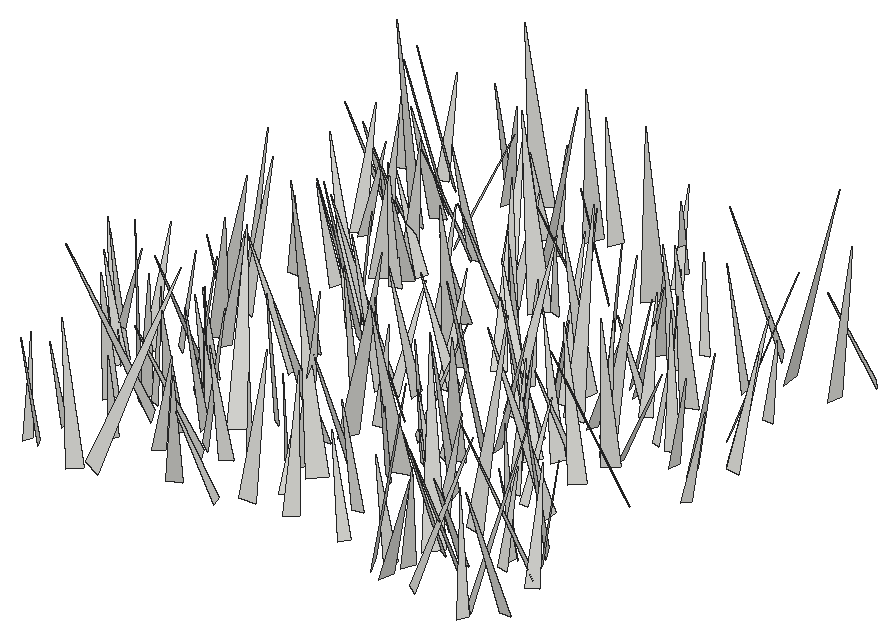
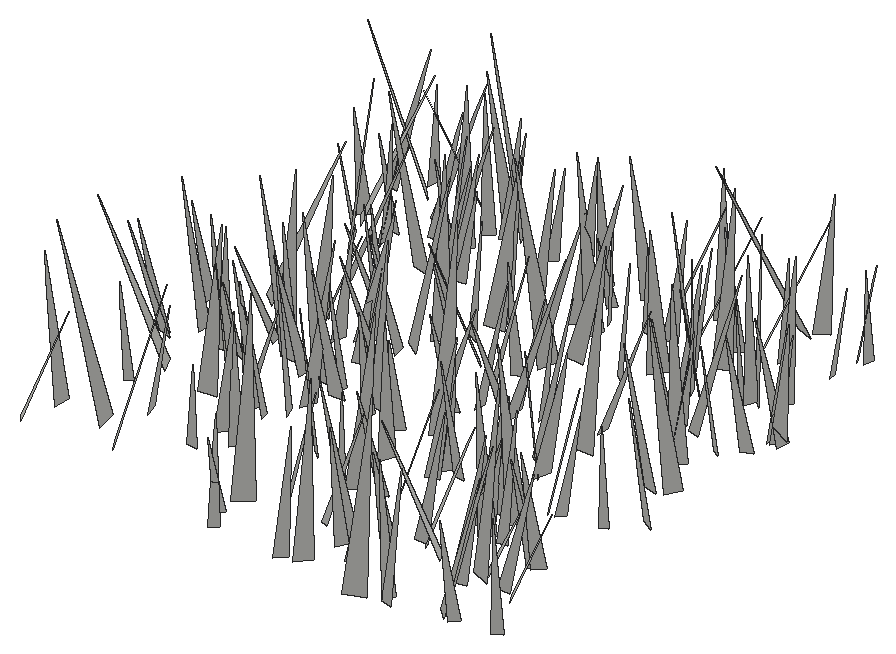
# SketchUp Ruby script. Lengths in inches.
U = 1.inch
M = Sketchup.active_model
def pt(a) = Geom::Point3d.new(a.map { |v| v * U })
def face(e, loops, mat)
  f = e.add_face(loops[0].map { |a| pt(a) })
  loops[1..].each { |l| e.add_face(l.map { |a| pt(a) }).erase! }
  f.material = f.back_material = mat if mat
  f
end
# faces: each face lists its corners as indices into pts; further lists are holes
def faces(e, pts, list, mat = nil) = list.each { |f| face(e, (f[0].is_a?(Array) ? f : [f]).map { |l| l.map { |i| pts[i] } }, mat) }
# xy, xz, yz: faces in a plane at the given z, y or x. An outline is a flat list of corners, or four numbers for a rectangle; further outlines are holes
def ring(l) = l.size == 4 ? [[l[0], l[1]], [l[2], l[1]], [l[2], l[3]], [l[0], l[3]]] : l.each_slice(2).to_a
def flat(e, list, mat, &to3) = list.each { |f| face(e, (f[0].is_a?(Array) ? f : [f]).map { |l| ring(l).map { |u, v| to3.(u, v) } }, mat) }
def xy(e, z, list, mat = nil) = flat(e, list, mat) { |x, y| [x, y, z] }
def xz(e, y, list, mat = nil) = flat(e, list, mat) { |x, z| [x, y, z] }
def yz(e, x, list, mat = nil) = flat(e, list, mat) { |y, z| [x, y, z] }
def lines(e, pts, list) = list.each { |a, b| e.add_line(pt(pts[a]), pt(pts[b])) }
# prism: a flat outline (further loops are holes) pulled along v
def prism(e, loops, v, mat = nil)
  f = face(e, loops, mat); d = Geom::Vector3d.new(v.map { |x| x * U })
  f.pushpull(f.normal.samedirection?(d) ? d.length : -d.length)
end
def box(e, o, s, mat = nil) = prism(e, [[o, [o[0] + s[0], o[1], o[2]], [o[0] + s[0], o[1] + s[1], o[2]], [o[0], o[1] + s[1], o[2]]]], [0, 0, s[2]], mat)
def at(x, y, z, deg = 0) = Geom::Transformation.translation(pt([x, y, z])) * Geom::Transformation.rotation(ORIGIN, Z_AXIS, deg.degrees)
def axes(o, x, y, z) = Geom::Transformation.new([*x, 0, *y, 0, *z, 0, *pt(o).to_a, 1])
def part(name) = M.definitions.add(name)
# library, detail: a bought-in or finely detailed component or shape, given as its bounding box
def library(name, o, s) = part(name).tap { |d| box(d.entities, o, s) }
def detail(e, o, s) = box(e.add_group.entities, o, s)
def put(e, d, t, mat = nil) = e.add_instance(d, t).tap { |i| i.material = mat if mat }
def group(e, t, mat = nil) = e.add_group.tap { |g| g.transformation = t; g.material = mat if mat }.entities
root = M.entities
c1 = part("fur_instance\#9")
p = [[0.8125,0,1.79],[0.67,-0.02,1.48],[0,-0.11,0],[0,0.11,0]]
faces(c1.entities,p,[[0,1,2,3]])
put(root,c1,axes([502.1875,404.34,-21.66],[2.0816,-3.74764,1.04429],[-3.88491,-2.06538,0.3318],[-0.20701,1.076,4.27408]))
put(root,c1,axes([503.84,370.23,-21.66],[3.17127,-3.30736,3.04126],[-3.82504,-3.9403,-0.2965],[-2.35731,1.94429,4.57249]))
put(root,c1,axes([504.64,399.73,-21.66],[-3.58425,-2.16039,0.18109],[-2.16614,3.55434,-0.47063],[-0.08907,0.49634,4.15845]))
put(root,c1,axes([504.66,370.01,-21.66],[-5.03296,-0.41167,1.23228],[-0.52474,5.15421,-0.42127],[1.18855,0.5323,5.03216]))
put(root,c1,axes([503.76,385.25,-21.66],[2.58353,5.00263,1.49189],[5.09313,-2.78069,0.50442],[-1.14546,-1.08079,5.60772]))
put(root,c1,axes([504.62,369.6,-21.66],[-3.50037,2.65675,1.28484],[2.86731,3.53339,0.50538],[0.69832,-1.19104,4.36526]))
put(root,c1,axes([503.45,370.17,-21.66],[4.85484,-0.93426,0.93937],[-1.01134,-4.91828,0.33525],[-0.85583,0.51221,4.93253]))
put(root,c1,axes([504.86,372.58,-21.66],[-0.99114,4.85366,1.48422],[5.00835,1.18049,-0.51592],[0.82303,-1.33855,4.92689]))
put(root,c1,axes([505.76,399.13,-21.66],[0.4513,-4.46287,0.47479],[-4.46772,-0.49211,-0.3789],[-0.42669,0.43236,4.4696]))
put(root,c1,axes([507.15,404.4375,-21.66],[2.82941,3.82153,3.56935],[4.50896,-3.83832,0.53527],[-2.64833,-2.45217,4.72474]))
put(root,c1,axes([506.2,356.96,-21.66],[-3.76859,1.24193,1.36163],[1.17189,4.00702,-0.41131],[1.42236,-0.01087,3.94658]))
put(root,c1,axes([505.79,395.09,-21.66],[-2.49427,4.27012,1.59064],[4.35584,2.76683,-0.59729],[1.33819,-1.04698,4.90903]))
put(root,c1,axes([505.79,404.8,-21.66],[2.7326,-2.75522,2.01665],[-3.2693,-2.85632,0.52755],[-0.98478,1.83723,3.84448]))
put(root,c1,axes([507.12,357.09,-21.66],[-3.57369,-1.9669,1.0397],[-2.0892,3.64317,-0.28897],[0.76478,0.76131,4.06896]))
put(root,c1,axes([505.91,387.55,-21.66],[0.58274,-3.68979,0.92218],[-3.78198,-0.46356,0.53511],[0.40205,0.98748,3.697]))
put(root,c1,axes([506.95,360.17,-21.66],[-3.35519,-0.75879,1.11745],[-0.66434,3.53232,0.40387],[1.17606,-0.1694,3.41613]))
put(root,c1,axes([508.16,397.96,-21.66],[-3.2308,-2.41105,0.08917],[-2.40238,3.20101,-0.49122],[-0.22293,0.4467,4.00124]))
put(root,c1,axes([505.3,380.38,-21.66],[5.59181,-3.37862,1.09906],[-3.46581,-5.63815,0.30113],[-0.78177,0.82912,6.52631]))
put(root,c1,axes([506.53,374.04,-21.66],[2.33806,3.32528,1.40975],[3.5899,-2.32407,-0.47188],[-0.3968,-1.43269,4.03749]))
put(root,c1,axes([506.39,395.07,-21.66],[3.89931,-1.45547,0.98195],[-1.58431,-3.9476,0.44006],[-0.75669,0.76505,4.13877]))
put(root,c1,axes([507.09,365.31,-21.66],[4.37094,-3.26497,1.75227],[-3.26747,-4.6741,-0.55863],[-1.74761,0.57306,5.42707]))
put(root,c1,axes([506.81,381.15,-21.66],[1.78136,5.8506,1.71123],[6.09225,-1.76893,-0.29408],[-0.20572,-1.72409,6.10871]))
put(root,c1,axes([508.73,401.61,-21.66],[-4.07714,-4.72232,1.18622],[-4.85623,4.056,-0.54439],[0.3528,1.25658,6.21506]))
put(root,c1,axes([507.76,377.96,-21.66],[-3.40624,-2.616,1.08161],[-2.59295,3.56228,0.44999],[1.13575,0.28715,4.27123]))
put(root,c1,axes([508.3125,398.65,-21.66],[-2.90002,-7.26429,3.03178],[-7.85451,2.88308,-0.60516],[0.51793,3.0479,7.79832]))
put(root,c1,axes([511.03,365.12,-21.66],[-6.73685,-3.71008,0.0403],[-3.70619,6.73292,0.28887],[0.17463,-0.23362,7.68547]))
put(root,c1,axes([508.9375,366.28,-21.66],[4.24793,5.0228,3.04998],[5.34423,-4.86703,0.57187],[-2.44337,-1.91294,6.55335]))
put(root,c1,axes([509.41,388.08,-21.66],[-3.58724,1.8714,1.40372],[2.1412,3.66165,0.59026],[0.94225,-1.19623,4.00275]))
put(root,c1,axes([508.99,400.3,-21.66],[1.67149,-5.33301,0.8085],[-5.34441,-1.75188,-0.5067],[-0.72935,0.6152,5.5658]))
put(root,c1,axes([507.59,376.98,-21.66],[3.73697,-5.4189,0.58942],[-5.45085,-3.71358,0.41766],[0.01126,0.72231,6.56925]))
put(root,c1,axes([509.49,372.86,-21.66],[-2.17037,-5.72704,0.1674],[-5.69455,2.17595,0.61228],[0.63178,-0.0613,6.09382]))
put(root,c1,axes([509,366.91,-21.66],[5.28351,-1.61661,1.62366],[-1.56193,-5.52709,-0.42043],[-1.67632,0.05465,5.50927]))
put(root,c1,axes([508.7,376.28,-21.66],[4.80209,-1.99507,1.20954],[-2.10711,-4.89697,0.2883],[-1.00169,0.73669,5.19204]))
put(root,c1,axes([510,366.68,-21.66],[1.76175,3.91399,1.38102],[4.01071,-1.99148,0.5277],[-1.06803,-1.02224,4.25965]))
put(root,c1,axes([510.51,388.11,-21.66],[-3.88391,-3.01754,1.00768],[-2.99103,4.00531,0.46572],[1.08383,0.24005,4.89626]))
put(root,c1,axes([510.1,393.9,-21.66],[0.02895,-4.95019,0.58964],[-4.94989,0.0415,0.59139],[0.59214,0.58889,4.91483]))
put(root,c1,axes([511.05,372.22,-21.66],[0.17752,-3.57602,1.3313],[-3.7929,-0.31113,-0.32997],[-0.41733,1.30655,3.56518]))
put(root,c1,axes([511.4,355.79,-21.66],[-3.51075,4.42455,2.16586],[4.8357,3.60279,0.47842],[0.94002,-2.00904,5.62789]))
put(root,c1,axes([511.19,405.79,-21.66],[-1.65824,-4.82946,1.36253],[-4.95542,1.80194,0.35604],[0.78993,1.16588,5.09379]))
put(root,c1,axes([510.89,360.84,-21.66],[3.12862,-2.29976,0.97047],[-2.27,-3.26853,-0.42753],[-1.03819,0.21622,3.85932]))
put(root,c1,axes([511.2,369.73,-21.66],[3.52114,3.87417,1.40413],[3.91467,-3.72163,0.45161],[-1.28689,-0.72073,5.21571]))
put(root,c1,axes([514.11,384.43,-21.66],[-6.63605,2.7216,0.19643],[2.70208,6.62626,-0.52374],[0.38006,0.41041,7.15332]))
put(root,c1,axes([513.33,392.98,-21.66],[-4.0044,1.49429,0.5536],[1.5481,4.00291,0.3933],[0.37782,-0.56428,4.25599]))
put(root,c1,axes([511.1,390.97,-21.66],[5.02607,-4.57327,2.19343],[-4.92834,-5.13329,0.59007],[-1.19892,1.92923,6.76964]))
put(root,c1,axes([512.8125,390.61,-21.66],[-0.34045,4.62028,2.07312],[5.05885,0.21591,0.34957],[-0.23002,-2.08976,4.6196]))
put(root,c1,axes([511.52,405.07,-21.66],[4.68677,-2.0034,0.66372],[-1.95488,-4.73014,-0.47351],[-0.79535,-0.17932,5.07496]))
put(root,c1,axes([511.71,393.625,-21.66],[3.13383,-5.16211,1.39491],[-5.34355,-3.08346,0.59403],[-0.19921,1.50298,6.00961]))
put(root,c1,axes([514.76,376.62,-21.66],[-5.6933,-0.47947,0.5538],[-0.44449,5.71072,0.37467],[0.58224,-0.32872,5.70116]))
put(root,c1,axes([514.36,397.34,-21.66],[-3.87512,-3.17972,0.32504],[-3.163,3.88842,0.32938],[0.4601,-0.04943,5.00187]))
put(root,c1,axes([513,391.81,-21.66],[2.62732,-3.98087,0.28129],[-3.95197,-2.64215,-0.47983],[-0.55532,-0.03119,4.74551]))
put(root,c1,axes([513.67,406.33,-21.66],[3.74176,-6.61768,2.63887],[-6.89022,-4.11933,-0.5604],[-1.81167,1.99888,7.58159]))
put(root,c1,axes([513.36,368.16,-21.66],[-4.21315,-2.34987,2.26772],[-2.4638,4.71684,0.31027],[2.14339,0.80291,4.81418]))
put(root,c1,axes([513.99,368.29,-21.66],[1.70929,-4.46495,1.67991],[-4.63149,-1.98085,-0.55231],[-1.1433,1.34907,4.74893]))
put(root,c1,axes([512.39,356.49,-21.66],[3.274,7.7332,0.0389],[7.72076,-3.26624,-0.49451],[0.44025,-0.22856,8.38313]))
put(root,c1,axes([513.92,379.8,-21.66],[-1.04012,-7.65192,1.88155],[-7.84849,1.17518,0.4406],[0.70237,1.80029,7.70971]))
put(root,c1,axes([514.86,397.1875,-21.66],[-0.19276,-5.01478,1.27598],[-5.16585,0.1124,-0.33865],[-0.30027,1.28555,5.00705]))
put(root,c1,axes([512.35,398.03,-21.66],[4.96423,2.67259,0.04648],[2.6631,-4.93667,-0.5706],[0.22978,-0.52435,5.60898]))
put(root,c1,axes([515.02,366.12,-21.66],[4.42222,0.57042,2.59632],[0.96066,-5.04183,-0.52855],[-2.47858,-0.93641,4.42741]))
put(root,c1,axes([513.71,364.26,-21.66],[4.30968,-5.09044,0.61484],[-5.06109,-4.35201,-0.55619],[-0.82219,0.10671,6.64655]))
put(root,c1,axes([515.69,383,-21.66],[-3.47477,-5.64058,1.59223],[-5.83486,3.50381,-0.32112],[0.55295,1.52727,6.61718]))
put(root,c1,axes([514.34,384.63,-21.66],[3.53151,3.08583,1.68165],[3.37882,-3.63698,-0.42174],[-0.96639,-1.43941,4.67077]))
put(root,c1,axes([517.29,363,-21.66],[-5.15654,-2.89646,0.02201],[-2.88562,5.14083,0.47427],[0.2514,-0.40276,5.89529]))
put(root,c1,axes([514.44,361.625,-21.66],[3.18493,-3.37138,0.77047],[-3.44968,-3.17103,0.3845],[-0.24394,0.82581,4.62191]))
put(root,c1,axes([516.98,367.53,-21.66],[-5.31707,5.30249,0.96243],[5.27581,5.39738,-0.58989],[1.09932,-0.2564,7.48596]))
put(root,c1,axes([517.04,398.32,-21.66],[-2.44616,4.11048,0.29857],[4.09909,2.46258,-0.31948],[0.42742,-0.0923,4.7726]))
put(root,c1,axes([516.91,402.79,-21.66],[1.11597,-3.30458,1.27259],[-3.40234,-1.37051,-0.57526],[-0.98175,0.99326,3.44016]))
put(root,c1,axes([516.77,363.96,-21.66],[3.29579,4.51514,1.8086],[4.80118,-3.36974,-0.33663],[-0.7786,-1.66678,5.57991]))
put(root,c1,axes([518.54,369.94,-21.66],[2.49829,3.83803,2.30798],[4.11646,-3.0089,0.54773],[-1.76409,-1.58579,4.54664]))
put(root,c1,axes([519.33,377.77,-21.66],[-4.34694,-0.07841,1.0456],[-0.20123,4.43859,-0.5037],[1.02905,0.53671,4.31837]))
put(root,c1,axes([520.95,379.48,-21.66],[-7.49054,-0.65717,0.9559],[-0.61994,7.54719,0.33069],[0.98046,-0.24861,7.51203]))
put(root,c1,axes([519.15,363.4,-21.66],[1.81609,-4.28388,1.69446],[-4.45246,-2.09973,-0.53642],[-1.18256,1.32684,4.62191]))
put(root,c1,axes([518.55,388.3125,-21.66],[0.78552,4.64999,1.51438],[4.88897,-0.70993,-0.35606],[0.11721,-1.55126,4.70241]))
put(root,c1,axes([520.07,393.28,-21.66],[-3.91317,-2.34388,0.53173],[-2.28614,3.94348,0.55853],[0.74167,-0.21123,4.52711]))
put(root,c1,axes([518.2,358.65,-21.66],[2.49567,-4.97649,0.70111],[-5.02561,-2.47346,0.33254],[-0.01412,0.77585,5.55727]))
put(root,c1,axes([518.94,401.16,-21.66],[-3.54773,2.23846,2.32232],[2.39169,4.14191,-0.33862],[2.16418,-0.90784,4.1812]))
put(root,c1,axes([521.25,378.35,-21.66],[-5.82181,0.2065,0.70872],[0.14567,5.84473,-0.50632],[0.72368,0.48471,5.80343]))
put(root,c1,axes([519.86,388.01,-21.66],[-3.10303,1.40825,1.48641],[1.65077,3.31728,0.3033],[1.21143,-0.91317,3.39411]))
put(root,c1,axes([519.69,404.64,-21.66],[-4.92901,3.2655,3.81824],[4.17297,5.6397,0.56365],[2.798,-2.65855,5.88565]))
put(root,c1,axes([519.32,399.61,-21.66],[6.35559,1.23086,1.81432],[1.1106,-6.60444,0.5901],[-1.89033,0.25813,6.44673]))
put(root,c1,axes([520.04,389.46,-21.66],[2.51881,-4.55482,0.15905],[-4.51842,-2.51942,-0.59372],[-0.59628,-0.14918,5.17091]))
put(root,c1,axes([522.31,358.3125,-21.66],[-4.25232,-1.15186,0.17503],[-1.13335,4.24309,0.38907],[0.27009,-0.33025,4.38835]))
put(root,c1,axes([521.24,363.55,-21.66],[1.02394,3.35387,1.44831],[3.57422,-1.23084,0.32333],[-0.75567,-1.27715,3.49176]))
put(root,c1,axes([521.26,405.23,-21.66],[-4.23654,2.45749,2.21286],[2.8358,4.54981,0.37637],[1.70124,-1.46429,4.88322]))
put(root,c1,axes([521.87,399.47,-21.66],[-2.1706,-3.79382,0.07549],[-3.76138,2.16267,0.53397],[0.50075,-0.20018,4.33814]))
put(root,c1,axes([521.2,393.61,-21.66],[0.22863,4.55848,1.01522],[4.65358,-0.13679,-0.43379],[0.39321,-1.03161,4.54355]))
put(root,c1,axes([523.23,394.08,-21.66],[-5.88987,4.84378,2.23578],[5.14185,6.04195,0.45575],[1.42207,-1.78441,7.61217]))
put(root,c1,axes([522.8,369.8125,-21.66],[-0.03159,-6.8611,0.78211],[-6.88005,-0.03586,-0.59249],[-0.59273,0.78192,6.83555]))
put(root,c1,axes([522.52,378.32,-21.66],[-0.04754,4.40868,0.34675],[4.41199,0.07095,-0.29716],[0.30179,-0.34273,4.39891]))
put(root,c1,axes([523.81,379.3125,-21.66],[-5.16901,0.01394,1.37798],[0.15537,5.32107,0.52899],[1.36927,-0.55116,5.14189]))
put(root,c1,axes([524.3,389.37,-21.66],[-5.32179,3.05618,1.70346],[3.04909,5.5718,-0.47069],[1.71611,-0.42222,6.11884]))
put(root,c1,axes([523.41,384.26,-21.66],[4.47344,-6.57845,1.38646],[-6.62258,-4.59864,-0.45163],[-1.15746,0.88686,7.94253]))
put(root,c1,axes([524.21,364.02,-21.66],[-3.74193,-1.93414,1.83822],[-1.95383,4.14237,0.38123],[1.81727,0.47108,4.19495]))
put(root,c1,axes([523.98,359.76,-21.66],[-0.55684,5.82392,2.02647],[6.12632,0.75415,-0.48394],[0.70204,-1.96161,5.83043]))
put(root,c1,axes([525.99,381.02,-21.66],[-4.59292,1.38597,0.57425],[1.45174,4.5724,0.57548],[0.37836,-0.71958,4.76284]))
put(root,c1,axes([525.14,376.16,-21.66],[-3.21192,-3.98216,0.77509],[-3.98629,3.28152,0.34045],[0.75355,0.38579,5.10471]))
put(root,c1,axes([524.18,394.57,-21.66],[-0.14412,-3.47359,1.04669],[-3.58722,0.2928,0.47779],[0.54152,1.01518,3.44359]))
put(root,c1,axes([523.99,366.04,-21.66],[6.73151,-1.98165,2.55494],[-2.23492,-7.11595,0.36912],[-2.33662,1.09735,7.00742]))
put(root,c1,axes([525.8125,365.48,-21.66],[-4.89648,5.17695,2.06152],[5.4889,4.95404,0.59637],[0.96057,-1.91907,7.10075]))
put(root,c1,axes([524.84,381.05,-21.66],[-1.136,4.49998,0.83575],[4.53043,1.22799,-0.4539],[0.65076,-0.69355,4.61891]))
put(root,c1,axes([524.62,374.03,-21.66],[-0.53957,3.97433,2.02364],[4.38519,0.84425,-0.48882],[0.81275,-1.91664,3.98089]))
put(root,c1,axes([526.11,398.31,-21.66],[-3.38614,-3.10021,1.02366],[-3.22386,3.40798,-0.34286],[0.51569,0.94841,4.57818]))
put(root,c1,axes([523.76,371.59,-21.66],[7.67247,-2.21843,2.0813],[-2.41925,-7.8734,0.52613],[-1.84403,1.09916,7.96941]))
put(root,c1,axes([525.47,362.12,-21.66],[-2.23531,2.8422,0.49749],[2.78374,2.28983,-0.57415],[0.75919,-0.0278,3.57002]))
put(root,c1,axes([526.26,385.63,-21.66],[-3.1637,4.01487,0.30871],[3.99884,3.17867,-0.35895],[0.47305,-0.01931,5.09895]))
put(root,c1,axes([526.73,368.25,-21.66],[-1.73362,-4.79917,0.85478],[-4.86621,1.65027,-0.60395],[-0.28757,1.00633,5.06683]))
put(root,c1,axes([527.8,360.01,-21.66],[3.60386,-3.42869,2.87422],[-4.08632,-4.02533,0.32181],[-1.82182,2.24626,4.96388]))
put(root,c1,axes([528.7,402.88,-21.66],[-2.71022,2.78687,0.60598],[2.7235,2.77712,-0.59105],[0.8464,-0.01233,3.84222]))
put(root,c1,axes([527.74,404.78,-21.66],[3.24769,-2.54753,0.32293],[-2.51539,-3.26077,-0.4265],[-0.51676,-0.13836,4.10555]))
put(root,c1,axes([528.51,400.43,-21.66],[5.1556,-5.75467,2.21602],[-5.90961,-5.43588,-0.36737],[-1.76168,1.39363,7.71761]))
put(root,c1,axes([529.75,368.61,-21.66],[-4.37552,-5.12362,2.64469],[-5.63456,4.50416,-0.59611],[1.22377,2.41912,6.71129]))
put(root,c1,axes([528.6875,391.9,-21.66],[4.00395,3.96639,1.91354],[4.25291,-4.1539,-0.28869],[-1.14309,-1.56151,5.62855]))
put(root,c1,axes([527.8,374.34,-21.66],[3.6626,3.70148,0.35684],[3.71844,-3.64024,-0.40601],[0.03906,-0.53912,5.19141]))
put(root,c1,axes([529.3,385.1875,-21.66],[-3.40994,2.09099,1.78678],[2.1335,3.80705,-0.3836],[1.73581,-0.57158,3.98156]))
put(root,c1,axes([529.52,384.1,-21.66],[1.75829,5.41715,3.42251],[6.36736,-1.87488,-0.30363],[-0.71818,-3.36006,5.68726]))
put(root,c1,axes([530.19,369.72,-21.66],[1.08245,-7.41016,1.80762],[-7.58562,-1.23679,-0.52762],[-0.7977,1.70574,7.47019]))
put(root,c1,axes([530.59,371.75,-21.66],[1.70203,4.17643,2.24286],[4.55719,-2.09788,0.44817],[-1.30578,-1.87783,4.48761]))
put(root,c1,axes([531.09,363.49,-21.66],[0.46643,-4.66615,1.44002],[-4.86096,-0.58186,-0.31092],[-0.46655,1.39737,4.67909]))
put(root,c1,axes([530.97,381.12,-21.66],[1.53253,6.73152,0.42824],[6.72346,-1.5597,0.45586],[-0.5402,-0.31526,6.8887]))
put(root,c1,axes([531.11,373.17,-21.66],[1.148,3.43718,0.90942],[3.54891,-1.0498,-0.51218],[0.21566,-1.0212,3.58745]))
put(root,c1,axes([532.92,375.65,-21.66],[-3.69542,-5.95234,1.80806],[-6.20183,3.68953,-0.52934],[0.48649,1.82006,6.98615]))
put(root,c1,axes([533.06,359.48,-21.66],[-3.14224,2.77876,1.0294],[2.91205,3.17344,0.32264],[0.54877,-0.92877,4.18224]))
put(root,c1,axes([532.63,384.59,-21.66],[-0.26987,6.47949,0.83868],[6.52839,0.23411,0.29205],[-0.25936,-0.84936,6.47853]))
put(root,c1,axes([533.54,386.73,-21.66],[-6.59669,1.20746,2.1658],[1.44471,6.87425,0.5679],[2.0153,-0.97558,6.6822]))
put(root,c1,axes([531.95,373.5625,-21.66],[2.97455,-6.14482,0.55918],[-6.16848,-2.94679,0.43089],[0.14598,0.69067,6.8133]))
put(root,c1,axes([536.25,376.92,-21.66],[-6.04879,4.39479,0.23194],[4.40071,6.03643,0.38865],[-0.04117,-0.45072,7.46666]))
put(root,c1,axes([533.01,383.41,-21.66],[4.24569,0.44069,0.96407],[0.53821,-4.32495,-0.39327],[-0.91322,-0.50013,4.25034]))
put(root,c1,axes([534.81,378.63,-21.66],[-5.38028,-3.08502,1.66928],[-3.07413,5.61908,0.47644],[1.68926,0.39986,6.18367]))
put(root,c1,axes([533.375,376.66,-21.66],[4.7353,0.6555,1.15241],[0.55235,-4.8611,0.49538],[-1.20525,0.34759,4.75472]))
put(root,c1,axes([534.83,383.51,-21.66],[-0.16365,8.04006,1.71484],[8.20749,0.06185,0.49328],[-0.46944,-1.72152,8.02659]))
put(root,c1,axes([535.16,369.51,-21.66],[-6.26815,-2.22604,2.13273],[-2.17784,6.6177,0.5065],[2.18193,0.21043,6.63238]))
put(root,c1,axes([533.94,388.42,-21.66],[5.56182,2.46032,2.03104],[2.73268,-5.78042,-0.48104],[-1.64644,-1.28288,6.06264]))
put(root,c1,axes([534.6,379.79,-21.66],[1.52104,-3.59534,0.18519],[-3.58042,-1.53172,-0.32978],[-0.37596,0.04131,3.88989]))
put(root,c1,axes([533.81,394.61,-21.66],[3.85722,-2.97975,0.1804],[-2.96484,-3.85827,-0.33622],[-0.3481,-0.15623,4.86251]))
put(root,c1,axes([536.03,393.59,-21.66],[-4.24357,2.27798,1.78244],[2.54082,4.44811,0.36434],[1.38223,-1.18292,4.80254]))
put(root,c1,axes([536.3,396.625,-21.66],[-0.50007,3.75556,1.02909],[3.87876,0.38868,0.46638],[-0.34425,-1.07612,3.75989]))
put(root,c1,axes([536.3,365.98,-21.66],[0.92533,-3.44435,1.34936],[-3.58141,-1.18238,-0.56215],[-0.92618,1.13092,3.52189]))
put(root,c1,axes([534.99,389.96,-21.66],[3.94564,1.0984,0.79467],[1.2,-3.96752,-0.47419],[-0.63087,-0.67703,4.06813]))
put(root,c1,axes([536.99,365.48,-21.66],[-4.76846,2.17787,1.48985],[2.383,4.8757,0.4998],[1.13316,-1.08876,5.21838]))
put(root,c1,axes([537.81,378.02,-21.66],[-5.43325,1.77797,0.85582],[1.73658,5.49897,-0.39929],[0.93695,0.1182,5.7028]))
put(root,c1,axes([537.94,387.88,-21.66],[-3.79704,-0.30553,0.54536],[-0.26679,3.82814,0.28712],[0.56533,-0.2455,3.79848]))
put(root,c1,axes([536.48,375.04,-21.66],[-2.09497,-3.98677,2.51489],[-4.46346,2.56262,0.34425],[1.51546,2.03632,4.49052]))
put(root,c1,axes([537.66,359.01,-21.66],[-3.6167,2.28369,2.19841],[2.80718,3.85669,0.61192],[1.47241,-1.74341,4.23336]))
put(root,c1,axes([536.8125,365.93,-21.66],[4.06657,-2.17936,1.39694],[-2.40276,-4.14574,0.52683],[-0.9632,1.14071,4.58356]))
put(root,c1,axes([539.01,362.3,-21.66],[-6.71454,4.39928,1.56364],[4.39375,6.8803,-0.4901],[1.57912,-0.43767,8.0124]))
put(root,c1,axes([538.4,365.12,-21.66],[-1.63509,-3.83691,0.93062],[-3.94815,1.58786,-0.39017],[-0.00453,1.00909,4.15248]))
put(root,c1,axes([536.19,389.2,-21.66],[5.46664,-0.56538,0.68203],[-0.51758,-5.49848,-0.40957],[-0.71898,-0.34055,5.48051]))
put(root,c1,axes([538.1875,372.46,-21.66],[0.28645,5.00767,1.03913],[5.08565,-0.389,0.47271],[-0.54104,-1.00525,4.99354]))
put(root,c1,axes([536.61,383.35,-21.66],[4.56446,-0.76979,0.5853],[-0.81155,-4.58493,0.29877],[-0.52586,0.39409,4.61927]))
put(root,c1,axes([536.8125,358.07,-21.66],[7.03431,3.48518,2.0857],[3.73576,-7.18871,-0.58711],[-1.59396,-1.46769,7.82836]))
put(root,c1,axes([539.54,378.08,-21.66],[-4.06839,-1.50308,0.30492],[-1.46625,4.06536,0.47647],[0.44983,-0.34301,4.31092]))
put(root,c1,axes([538.57,387.01,-21.66],[-3.00951,3.51493,1.30262],[3.55292,3.20728,-0.44587],[1.1951,-0.68362,4.60577]))
put(root,c1,axes([539.73,362.48,-21.66],[-2.91722,-4.26379,0.81225],[-4.33997,2.88016,-0.46811],[0.06569,0.93518,5.14499]))
put(root,c1,axes([539.22,388.68,-21.66],[-4.16278,-2.64249,2.71758],[-3.23685,4.57857,-0.50613],[1.97251,1.93665,4.90462]))
put(root,c1,axes([542.33,371.43,-21.66],[-7.29173,-1.24054,0.1592],[-1.24954,7.26646,-0.60898],[0.05425,0.6271,7.37139]))
put(root,c1,axes([540.73,399.93,-21.66],[-5.52316,-3.7636,0.965],[-3.71814,5.60658,0.58551],[1.12752,0.05244,6.65787]))
put(root,c1,axes([539.45,366.4375,-21.66],[1.82525,7.99707,1.79582],[8.16577,-1.93273,0.30716],[-0.70587,-1.67961,8.19697]))
put(root,c1,axes([538.85,382.38,-21.66],[1.36969,7.27883,2.41401],[7.66649,-1.2409,-0.6083],[0.18385,-2.48268,7.38156]))
put(root,c1,axes([539.82,371.54,-21.66],[0.7,4.04155,0.09862],[4.02713,-0.70587,0.34334],[-0.35517,-0.03822,4.08733]))
put(root,c1,axes([540.14,380.41,-21.66],[0.9151,5.15761,1.58711],[5.35443,-1.06795,0.38322],[-0.67079,-1.48856,5.22413]))
put(root,c1,axes([540.22,389.95,-21.66],[1.19646,-6.35488,2.45253],[-6.76034,-1.41301,-0.36331],[-0.83491,2.33448,6.45631]))
put(root,c1,axes([538.95,359.42,-21.66],[4.27597,-2.96302,0.67606],[-2.94629,-4.32773,-0.33261],[-0.74558,0.10858,5.19161]))
put(root,c1,axes([540.88,376.3,-21.66],[3.04965,-4.5466,3.26672],[-5.09549,-3.79519,-0.52522],[-2.31926,2.35973,5.44941]))
put(root,c1,axes([538.67,357.3,-21.66],[5.31861,-1.95589,0.12332],[-1.94358,-5.30997,-0.39374],[-0.25139,-0.32717,5.65315]))
put(root,c1,axes([541.83,394.3,-21.66],[-4.7779,-0.84592,1.0787],[-0.97294,4.84801,-0.50762],[0.9657,0.69908,4.82558]))
put(root,c1,axes([541.17,379.76,-21.66],[-3.30956,4.62511,3.28339],[5.43338,3.67626,0.29816],[1.62808,-2.86687,5.67942]))
put(root,c1,axes([541.65,384.35,-21.66],[1.21689,3.56799,0.58582],[3.55761,-1.29191,0.47847],[-0.64586,-0.39367,3.73931]))
put(root,c1,axes([541.75,362.31,-21.66],[-0.76321,-4.71965,0.1503],[-4.6984,0.77422,0.45372],[0.47201,0.07524,4.75939]))
put(root,c1,axes([543.2,360.33,-21.66],[-2.96525,-5.05492,0.58848],[-5.08807,2.93137,-0.45808],[-0.10025,0.73898,5.84252]))
put(root,c1,axes([541.26,357.01,-21.66],[3.77289,4.9439,0.17652],[4.9129,-3.7705,0.5956],[-0.58026,0.22179,6.19049]))
put(root,c1,axes([541.2,380.86,-21.66],[3.9948,0.59542,0.26899],[0.55235,-3.96784,0.58004],[-0.34899,0.53573,3.99706]))
put(root,c1,axes([543.22,384.2,-21.66],[-1.15441,5.11883,1.74969],[5.40957,1.09949,0.35248],[0.0216,-1.78472,5.23554]))
put(root,c1,axes([545.29,376.49,-21.66],[-4.1792,-5.61615,0.15739],[-5.61189,4.16336,-0.45249],[-0.26934,0.3962,6.98585]))
put(root,c1,axes([544.18,364.6,-21.66],[-5.10853,0.04095,1.59169],[-0.11644,5.32521,-0.51071],[1.58796,0.52222,5.08311]))
put(root,c1,axes([544.28,365.1875,-21.66],[-2.57629,-2.49445,0.93197],[-2.62206,2.60252,-0.28257],[0.46438,0.85602,3.57488]))
put(root,c1,axes([544.4,363.32,-21.66],[0.69151,3.97199,1.28395],[4.17346,-0.6309,-0.296],[0.08642,-1.31479,4.02085]))
put(root,c1,axes([543.33,397.54,-21.66],[8.05424,1.38868,1.7961],[1.29513,-8.24767,0.56905],[-1.86468,0.26973,8.15325]))
put(root,c1,axes([547.45,363.36,-21.66],[-5.40162,-4.18627,0.13743],[-4.18531,5.38577,-0.4449],[-0.16419,0.43574,6.81941]))
put(root,c1,axes([545.53,367.05,-21.66],[-5.52938,-3.456,2.07939],[-3.45701,5.87854,0.57763],[2.07771,0.58365,6.49494]))
put(root,c1,axes([544.66,382.64,-21.66],[4.24921,-1.39082,0.67887],[-1.35455,-4.30166,-0.33452],[-0.74864,-0.11098,4.4585]))
put(root,c1,axes([546.67,356.02,-21.66],[-4.5869,1.43943,1.05541],[1.33614,4.69877,-0.60151],[1.18347,0.27406,4.76967]))
put(root,c1,axes([545.76,391.93,-21.66],[0.94774,-3.5048,1.15841],[-3.67796,-0.79512,0.60341],[0.31324,1.26803,3.58018]))
put(root,c1,axes([546.32,365.4375,-21.66],[3.3556,2.16226,1.21696],[2.08771,-3.56664,0.58052],[-1.34083,-0.14202,3.94948]))
put(root,c1,axes([545.04,388.46,-21.66],[6.72288,3.05704,0.61475],[3.02645,-6.7488,0.46346],[-0.75102,0.16938,7.37074]))
put(root,c1,axes([548.42,401.01,-21.66],[-3.47143,-2.84551,0.09651],[-2.81271,3.45107,0.57956],[0.4415,-0.38766,4.45106]))
put(root,c1,axes([546.2,357.43,-21.66],[5.62974,5.25868,1.12192],[5.27805,-5.71471,0.30107],[-1.02693,-0.54292,7.69786]))
put(root,c1,axes([546.27,382.6875,-21.66],[5.73568,-0.06882,1.05766],[0.01363,-5.81521,-0.45231],[-1.05981,-0.44725,5.71823]))
put(root,c1,axes([547.81,362.52,-21.66],[-2.87037,3.7349,1.34525],[3.80013,3.06525,-0.40189],[1.14815,-0.80807,4.69329]))
put(root,c1,axes([547.53,397.39,-21.66],[5.90361,-0.69248,2.28384],[-0.937,-6.27702,0.51884],[-2.19488,0.81708,5.9214]))
put(root,c1,axes([548.74,358.27,-21.66],[-0.82643,-5.48525,0.94931],[-5.54864,0.73423,-0.58792],[-0.44918,1.02229,5.51591]))
put(root,c1,axes([548.03,385.02,-21.66],[1.54833,5.59255,0.52827],[5.59137,-1.58705,0.41342],[-0.54067,-0.39706,5.78818]))
put(root,c1,axes([548.37,384.72,-21.66],[0.17579,4.7582,1.26729],[4.89735,-0.03702,-0.54033],[0.51227,-1.27889,4.73069]))
put(root,c1,axes([548.55,379.15,-21.66],[3.49135,-1.63355,1.08284],[-1.80913,-3.53699,0.49727],[-0.7537,0.9229,3.8224]))
